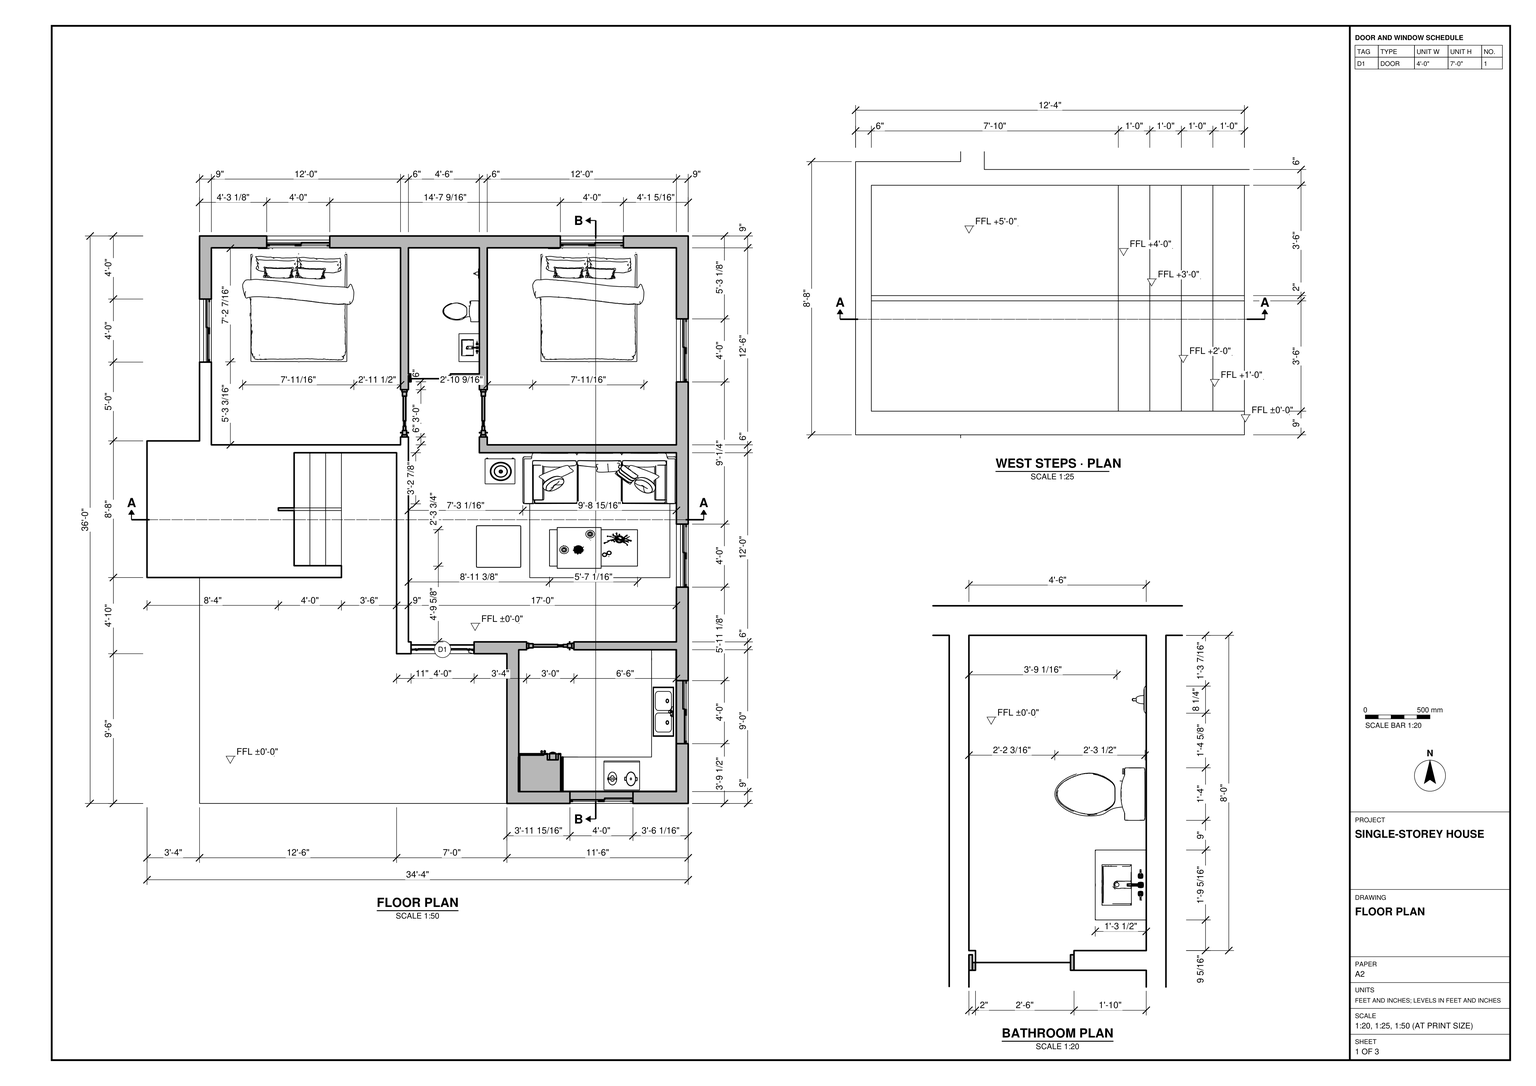
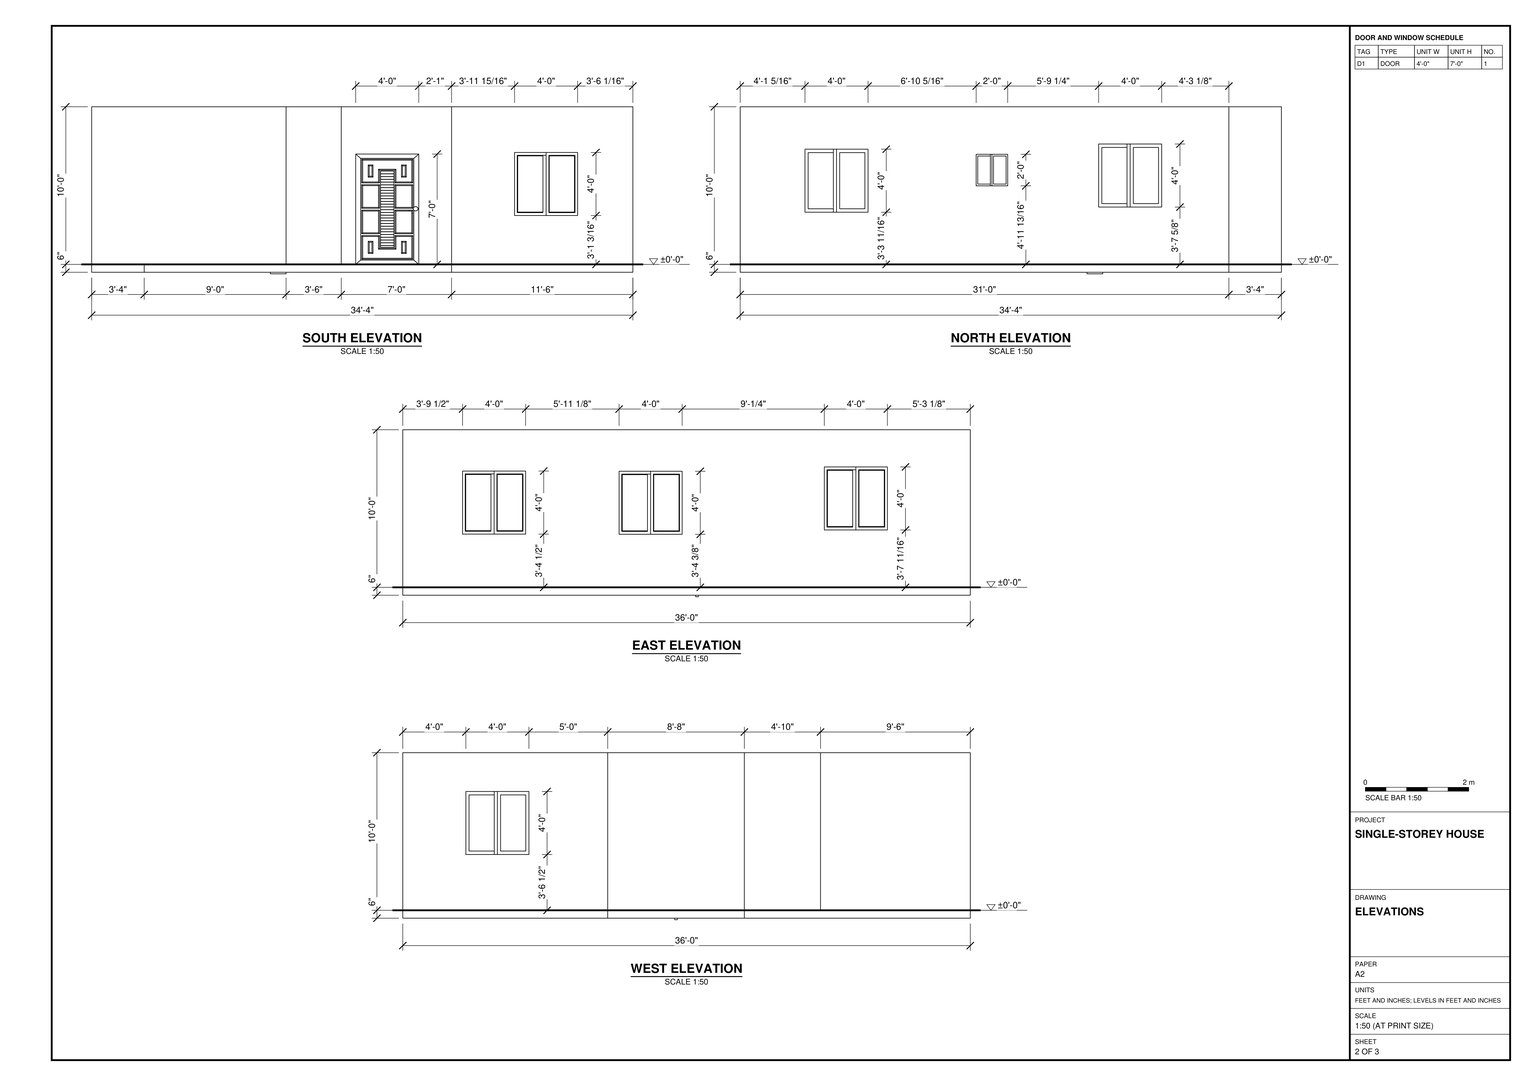
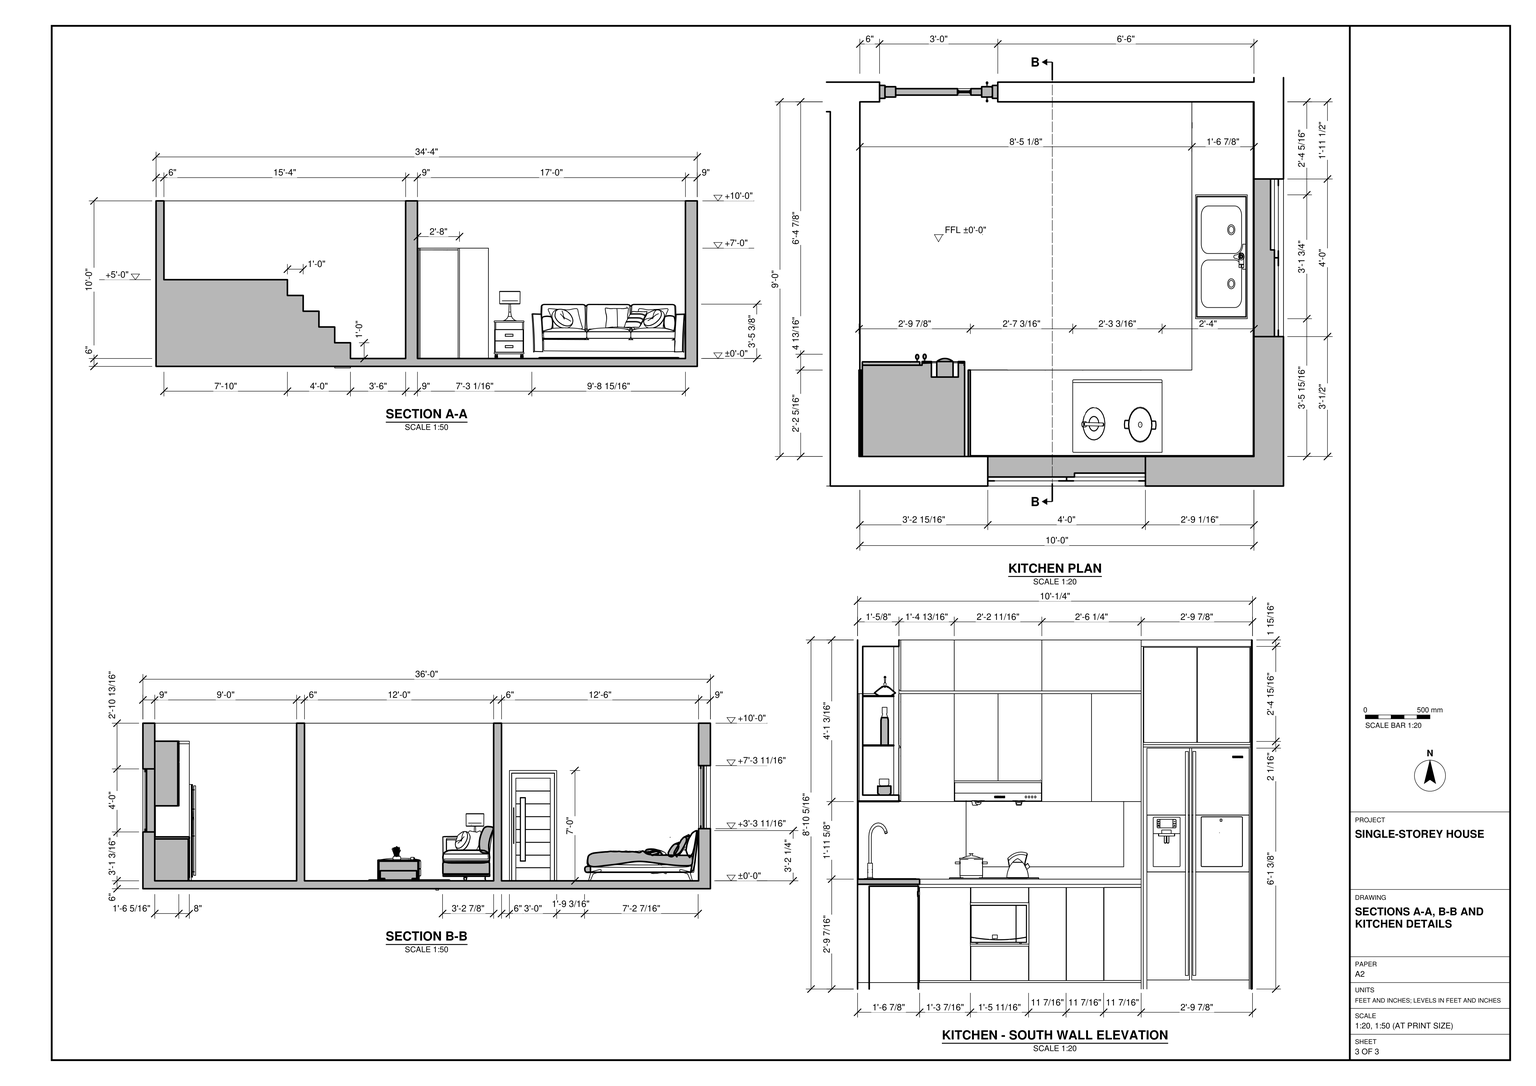
Build the house in SketchUp from task_files/diagram_01.pdf. Work in feet and inches. Set the finished floor of the single storey at ±0'-0". The overall model, including the west steps and floor slab, is 34'-4" east to west, 36'-0" north to south and 10'-7 3/16" high.

Follow the stepped footprint in the floor plan. Place the two bedrooms across the north end, with the narrow bathroom between them, the living room to the south and the kitchen projecting at the southeast corner. Model the 6" floor slab and use the wall thicknesses marked on the plan, including the 9" exterior walls and 6" partitions where indicated. Follow the level wall tops in the elevations. Use the enlarged west steps plan and section A-A to set out the raised landing and its flight down towards the house.

Fit the south entrance door and place the windows at the offsets and sill heights shown in the elevations. Position the beds, sofa and tables to match their plan footprints. Fit the bathroom toilet and vanity against the east wall. Use the kitchen detail views for the counters, lower and upper cabinets, sink, cooktop and refrigerator. Decor and loose items, including appliances, may be any suitable library components.

Keep shell elements and each furniture or joinery piece in separate groups or components, and use components for repeated parts. Save one SketchUp model as output_files/single_storey_house_with_west_steps_and_fitted_kitchen.skp.

# SketchUp Ruby script. Lengths in inches.
U = 1.inch
M = Sketchup.active_model
def pt(a) = Geom::Point3d.new(a.map { |v| v * U })
def face(e, loops, mat)
  f = e.add_face(loops[0].map { |a| pt(a) })
  loops[1..].each { |l| e.add_face(l.map { |a| pt(a) }).erase! }
  f.material = f.back_material = mat if mat
  f
end
# faces: each face lists its corners as indices into pts; further lists are holes
def faces(e, pts, list, mat = nil) = list.each { |f| face(e, (f[0].is_a?(Array) ? f : [f]).map { |l| l.map { |i| pts[i] } }, mat) }
# xy, xz, yz: faces in a plane at the given z, y or x. An outline is a flat list of corners, or four numbers for a rectangle; further outlines are holes
def ring(l) = l.size == 4 ? [[l[0], l[1]], [l[2], l[1]], [l[2], l[3]], [l[0], l[3]]] : l.each_slice(2).to_a
def flat(e, list, mat, &to3) = list.each { |f| face(e, (f[0].is_a?(Array) ? f : [f]).map { |l| ring(l).map { |u, v| to3.(u, v) } }, mat) }
def xy(e, z, list, mat = nil) = flat(e, list, mat) { |x, y| [x, y, z] }
def xz(e, y, list, mat = nil) = flat(e, list, mat) { |x, z| [x, y, z] }
def yz(e, x, list, mat = nil) = flat(e, list, mat) { |y, z| [x, y, z] }
def lines(e, pts, list) = list.each { |a, b| e.add_line(pt(pts[a]), pt(pts[b])) }
# prism: a flat outline (further loops are holes) pulled along v
def prism(e, loops, v, mat = nil)
  f = face(e, loops, mat); d = Geom::Vector3d.new(v.map { |x| x * U })
  f.pushpull(f.normal.samedirection?(d) ? d.length : -d.length)
end
def box(e, o, s, mat = nil) = prism(e, [[o, [o[0] + s[0], o[1], o[2]], [o[0] + s[0], o[1] + s[1], o[2]], [o[0], o[1] + s[1], o[2]]]], [0, 0, s[2]], mat)
def at(x, y, z, deg = 0) = Geom::Transformation.translation(pt([x, y, z])) * Geom::Transformation.rotation(ORIGIN, Z_AXIS, deg.degrees)
def axes(o, x, y, z) = Geom::Transformation.new([*x, 0, *y, 0, *z, 0, *pt(o).to_a, 1])
def part(name) = M.definitions.add(name)
# library, detail: a bought-in or finely detailed component or shape, given as its bounding box
def library(name, o, s) = part(name).tap { |d| box(d.entities, o, s) }
def detail(e, o, s) = box(e.add_group.entities, o, s)
def put(e, d, t, mat = nil) = e.add_instance(d, t).tap { |i| i.material = mat if mat }
def group(e, t, mat = nil) = e.add_group.tap { |g| g.transformation = t; g.material = mat if mat }.entities
root = M.entities
M.materials.add("Polis06_194").color = [79, 50, 36]
M.materials.add("[0012_Bisque]").color = [255, 228, 196]
M.materials.add("[Blacktop Old 02]").color = [143, 145, 145]
M.materials.add("[Carrera Marble]").color = [207, 207, 207]
M.materials.add("[Color M00]1").color = [255, 255, 255]
M.materials.add("[Color M05]").color = [100, 98, 98]
M.materials.add("[Color M07]").color = [46, 46, 46]
M.materials.add("[Color_001]").color = [226, 226, 226]
M.materials.add("[Field Square Tile]").color = [217, 201, 169]
M.materials.add("[Metal_Corrogated_Shiny]").color = [126, 127, 128]
M.materials.add("[Metal_Corrogated_Shiny]1").color = [193, 193, 193]
M.materials.add("[Translucent Glass Blue]").color = [100, 149, 237]
M.materials["[Translucent Glass Blue]"].alpha = 0.5
M.materials.add("[_0030_OldLace_]").color = [200, 200, 200]
M.materials.add("行者0155_1_1").color = [98, 90, 80]
c1 = library("devendra+jangid+[door]+drawings",[57.04,80.03,0],[48,84,6.66])
c2 = library("Спалня Венид",[0.07,-0.07,0],[84.71,86.8,39])
c3 = library("04+Sofa+y+Mesas (1)",[-94.93,-111.67,3.93],[153.81,110.61,64.28])
c4 = part("Janela aluminio")
xy(c4.entities,0,[[0,0,47.24,1.57],[23.62,1.57,47.24,2.76],[0,2.76,25.98,3.9375],[0,3.9375,47.24,5.91]])
xy(c4.entities,43.31,[[0,0,47.24,1.57],[23.62,1.57,47.24,2.76],[0,2.76,0,5.91,47.24,5.91,47.24,3.9375,25.98,3.9375,25.98,2.76],[25.98,2.76,47.24,3.9375]])
xz(c4.entities,1.57,[[0,0,23.62,0,23.62,41.34,21.26,41.34,21.26,1.97,1.97,1.97,1.97,41.34,23.62,41.34,23.62,43.31,0,43.31],[[23.62,0,47.24,43.31],[25.7,1.97,45.28,41.34]]])
xz(c4.entities,2.76,[[[0,0,23.62,43.31],[2.36,2.36,21.26,40.94]],[23.62,0,25.98,43.31]])
xz(c4.entities,2.76,[[2.36,2.36,21.26,40.94]],"[Translucent Glass Blue]")
xz(c4.entities,3.9375,[[25.98,0,25.98,2.36,44.88,2.36,44.88,40.94,25.98,40.94,25.98,43.31,47.24,43.31,47.24,0]])
xz(c4.entities,3.9375,[[25.98,2.36,44.88,40.94]],"[Translucent Glass Blue]")
yz(c4.entities,0,[[0,0,1.57,43.31],[2.76,0,5.91,43.31]])
yz(c4.entities,23.62,[[1.57,0,2.76,43.31]])
yz(c4.entities,25.98,[[2.76,0,3.9375,43.31]])
yz(c4.entities,47.24,[[0,0,1.57,43.31],[1.57,0,2.76,43.31],[3.9375,0,5.91,43.31]])
c5 = library("Framed entrance door",[0,0,0],[5.9375,43.31,84.65])
c6 = part("群组\#3")
xy(c6.entities,0,[[0,0,4.72,1.18],[0,34.25,4.72,35.43]],"Polis06_194")
xy(c6.entities,85.26,[[0,1.18,4.72,34.25]],"Polis06_194")
xy(c6.entities,86.61,[[0,0,4.72,35.43]],"Polis06_194")
xz(c6.entities,0,[[0,0,4.72,86.61]],"Polis06_194")
xz(c6.entities,1.18,[[0,0,2.36,85.26],[2.36,0,4.72,85.26]],"Polis06_194")
xz(c6.entities,34.25,[[0,0,4.72,85.26]],"Polis06_194")
xz(c6.entities,35.43,[[0,0,4.72,86.61]],"Polis06_194")
yz(c6.entities,0,[[0,0,1.18,86.61],[34.25,0,35.43,86.61],[1.18,85.26,34.25,86.61]],"Polis06_194")
yz(c6.entities,2.36,[[1.18,0,34.25,0,34.25,85.21,1.18,85.26]],"Polis06_194")
yz(c6.entities,4.72,[[0,0,1.18,86.61],[34.25,0,35.43,86.61],[1.18,85.26,34.25,86.61]],"Polis06_194")
c7 = library("TS396-4",[-0.02,-3.5,-3.5],[8.95,7,28.74])
c8 = library("K-3457 - Kohler Devonshire(R) elongated toilet with left-han",[-8.99,-6.22,0],[17.99,30.87,31.5])
c9 = library("30\" Kohler Jacquard Vanity",[0,0,0],[30,21.875,40.63])
c10 = part("Dishwasher5")
xy(c10.entities,0,[[0.39,0,29.13,23.62]],"[Metal_Corrogated_Shiny]")
xy(c10.entities,35.45,[[0.39,0,29.13,0.39]])
xy(c10.entities,35.49,[[0.39,0,29.13,0.39]])
xy(c10.entities,35.81,[[12.33,0,17.95,0.39]])
xy(c10.entities,37.36,[[12.33,0,17.95,0.39]])
xy(c10.entities,39.37,[[0.39,0,29.13,23.62]],"[Metal_Corrogated_Shiny]")
xz(c10.entities,-0.39,[[6.875,36.35,7.125,36.38,7.36,36.48,7.5625,36.63,7.72,36.84,7.82,37.08,7.86,37.34,7.83,37.59,7.74,37.84,7.59,38.05,7.39,38.21,7.16,38.32,6.91,38.35,6.66,38.33,6.43,38.23,6.22,38.07,6.06,37.87,5.96,37.63,5.93,37.375,5.95,37.11,6.05,36.87,6.2,36.66,6.39,36.5,6.625,36.39]],"[Metal_Corrogated_Shiny]1")
xz(c10.entities,0,[[0.39,0,29.13,35.45],[[0.39,35.49,29.13,39.37],[12.33,35.81,17.95,37.36],[6.875,36.35,6.625,36.39,6.39,36.5,6.2,36.66,6.05,36.87,5.95,37.11,5.93,37.375,5.96,37.63,6.06,37.87,6.22,38.07,6.43,38.23,6.66,38.33,6.91,38.35,7.16,38.32,7.39,38.21,7.59,38.05,7.74,37.84,7.83,37.59,7.86,37.34,7.82,37.08,7.72,36.84,7.5625,36.63,7.36,36.48,7.125,36.38]]])
xz(c10.entities,0.39,[[0.39,35.45,29.13,35.49],[12.33,35.81,17.95,37.36]])
xz(c10.entities,23.62,[[0.39,0,29.13,39.37]],"[Metal_Corrogated_Shiny]")
yz(c10.entities,0.39,[[0,0,0,35.45,0.39,35.45,0.39,35.49,0,35.49,0,39.37,23.62,39.37,23.62,0]],"[Metal_Corrogated_Shiny]")
yz(c10.entities,12.33,[[0,35.81,0.39,37.36]])
yz(c10.entities,17.95,[[0,35.81,0.39,37.36]])
yz(c10.entities,29.13,[[0,0,23.62,0,23.62,39.37,0,39.37,0,35.49,0.39,35.49,0.39,35.45,0,35.45]],"[Metal_Corrogated_Shiny]")
p = [[6.39,0,36.5],[6.625,0,36.39],[6.625,-0.39,36.39],[6.39,-0.39,36.5],[6.875,0,36.35],[6.875,-0.39,36.35],
  [7.125,0,36.38],[7.125,-0.39,36.38],[7.36,0,36.48],[7.36,-0.39,36.48],[6.2,0,36.66],[6.2,-0.39,36.66],
  [7.5625,0,36.63],[7.5625,-0.39,36.63],[7.72,0,36.84],[7.72,-0.39,36.84],[6.05,0,36.87],[6.05,-0.39,36.87],
  [7.82,0,37.08],[7.82,-0.39,37.08],[5.95,0,37.11],[5.95,-0.39,37.11],[5.93,0,37.375],[5.93,-0.39,37.375],
  [7.86,0,37.34],[7.86,-0.39,37.34],[7.83,0,37.59],[7.83,-0.39,37.59],[5.96,0,37.63],[5.96,-0.39,37.63],
  [6.06,0,37.87],[6.06,-0.39,37.87],[7.74,0,37.84],[7.74,-0.39,37.84],[7.59,0,38.05],[7.59,-0.39,38.05],
  [6.22,0,38.07],[6.22,-0.39,38.07],[7.39,0,38.21],[7.39,-0.39,38.21],[6.43,0,38.23],[6.43,-0.39,38.23],
  [6.66,0,38.33],[6.66,-0.39,38.33],[7.16,0,38.32],[7.16,-0.39,38.32],[6.91,0,38.35],[6.91,-0.39,38.35]]
faces(c10.entities,p,[[0,1,2,3],[1,4,5,2],[4,6,7,5],[6,8,9,7],[10,0,3,11],[8,12,13,9],[12,14,15,13],[16,10,11,17],
  [14,18,19,15],[20,16,17,21],[22,20,21,23],[18,24,25,19],[24,26,27,25],[28,22,23,29],[30,28,29,31],[26,32,33,27],
  [32,34,35,33],[36,30,31,37],[34,38,39,35],[40,36,37,41],[42,40,41,43],[38,44,45,39],[46,42,43,47],[44,46,47,45]],"[Metal_Corrogated_Shiny]1")
c11 = library("1",[-25.2,23.2,0],[33.86,19.68,25.36])
c12 = part("Cabinet panel \#1")
xy(c12.entities,0,[[0.6,0.08,0.63,16.59]],"行者0155_1_1")
xy(c12.entities,27.1,[[0.08,0.08,0.63,16.59]],"行者0155_1_1")
xz(c12.entities,0,[[0.52,0.08,0.63,0.08,0.63,27.02,0.08,27.02,0.08,0.53]],"行者0155_1_1")
xz(c12.entities,16.67,[[0.52,0.08,0.08,0.53,0.08,27.02,0.63,27.02,0.63,0.08]],"行者0155_1_1")
yz(c12.entities,0,[[0.08,0.61,16.59,27.02]],"行者0155_1_1")
yz(c12.entities,0.71,[[0.08,0.08,16.59,27.02]],"行者0155_1_1")
p = [[0.41,0.08,0.08],[0.6,0.08,0],[0.52,0,0.08],[0.63,0,0.08],[0.63,0.08,0],[0.71,0.08,0.08],
  [0.41,16.59,0.08],[0.6,16.59,0],[0.71,16.59,0.08],[0.63,16.59,0],[0.52,16.67,0.08],[0.63,16.67,0.08],
  [0.08,0.08,0.42],[0.08,0,0.53],[0.71,0.08,27.02],[0.63,0,27.02],[0.08,16.59,0.42],[0.08,16.67,0.53],
  [0.71,16.59,27.02],[0.63,16.67,27.02],[0,0.08,0.61],[0,16.59,0.61],[0,0.08,27.02],[0.08,0,27.02],
  [0,16.59,27.02],[0.08,16.67,27.02],[0.08,0.08,27.1],[0.63,0.08,27.1],[0.08,16.59,27.1],[0.63,16.59,27.1]]
faces(c12.entities,p,[[0,1,2],[3,2,1,4],[4,5,3],[0,6,7,1],[8,5,4,9],[7,6,10],[10,11,9,7],[8,9,11],
  [12,0,2,13],[5,14,15,3],[0,12,16,6],[6,16,17,10],[18,8,11,19],[20,12,13],[16,12,20,21],[16,21,17],
  [22,20,13,23],[21,24,25,17],[26,22,23],[27,26,23,15],[14,27,15],[26,28,24,22],[29,27,14,18],[24,28,25],
  [28,29,19,25],[29,18,19]],"行者0155_1_1")
c13 = library("Range hood",[0,0.31,0],[20.46,27.69,6.07])
c14 = part("Component\#6")
prism(c14.entities,[[[0,0,0],[0,0,28.41],[0,0.53,28.9375],[0,0.71,28.9375],[0,0.71,0]]],[17.47,0,0],"行者0155_1_1")
c15 = part("Cabinet panel \#2")
xy(c15.entities,0,[[0.63,0.079,0.641,18.822]],"行者0155_1_1")
xy(c15.entities,32.864,[[0.079,0.079,0.63,18.822]],"行者0155_1_1")
xz(c15.entities,0,[[0.5625,0.079,0.63,0.079,0.63,32.786,0.079,32.786,0.079,0.5625]],"行者0155_1_1")
xz(c15.entities,18.9,[[0.5625,0.079,0.079,0.5625,0.079,32.786,0.63,32.786,0.63,0.079]],"行者0155_1_1")
yz(c15.entities,0,[[0.079,0.641,18.822,32.786]],"行者0155_1_1")
yz(c15.entities,0.709,[[0.079,0.079,18.822,32.786]],"行者0155_1_1")
p = [[0.633,0.079,0.003],[0.641,0.079,0],[0.63,0.068,0.011],[0.5625,0,0.079],[0.451,0.079,0.079],[0.63,0.079,0],
  [0.63,0,0.079],[0.709,0.079,0.079],[0.641,18.822,0],[0.451,18.822,0.079],[0.633,18.822,0.003],[0.63,18.822,0],
  [0.709,18.822,0.079],[0.63,18.833,0.011],[0.5625,18.9,0.079],[0.63,18.9,0.079],[0.079,0.079,0.451],[0.079,0,0.5625],
  [0.709,0.079,32.786],[0.63,0,32.786],[0.079,18.822,0.451],[0.079,18.9,0.5625],[0.709,18.822,32.786],[0.63,18.9,32.786],
  [0,0.079,0.641],[0,18.822,0.641],[0,0.079,32.786],[0.079,0,32.786],[0,18.822,32.786],[0.079,18.9,32.786],
  [0.079,0.079,32.864],[0.63,0.079,32.864],[0.079,18.822,32.864],[0.63,18.822,32.864]]
faces(c15.entities,p,[[0,1,2,3,4],[1,5,2,6,3,2],[5,0,7,6,2],[8,1,0,4,9,10],[5,11,10,12,7,0],[13,8,10,9,14],[10,11,13,15,12],[11,8,13,14,15,13],
  [16,4,3,17],[7,18,19,6],[16,20,9,4],[21,14,9,20],[22,12,15,23],[24,16,17],[20,16,24,25],[20,25,21],
  [26,24,17,27],[25,28,29,21],[30,26,27],[31,30,27,19],[18,31,19],[30,32,28,26],[33,31,18,22],[28,32,29],
  [32,33,23,29],[33,22,23]],"行者0155_1_1")
c16 = part("Cabinet panel \#3")
xy(c16.entities,0,[[0.6,0.08,0.63,16.59]],"行者0155_1_1")
xy(c16.entities,27.1,[[0.08,0.08,0.63,16.59]],"行者0155_1_1")
xz(c16.entities,0,[[0.52,0.08,0.63,0.08,0.63,27.02,0.08,27.02,0.08,0.53]],"行者0155_1_1")
xz(c16.entities,16.67,[[0.52,0.08,0.08,0.53,0.08,27.02,0.63,27.02,0.63,0.08]],"行者0155_1_1")
yz(c16.entities,0,[[0.08,0.61,16.59,27.02]],"行者0155_1_1")
yz(c16.entities,0.71,[[0.08,0.08,16.59,27.02]],"行者0155_1_1")
p = [[0.41,0.08,0.08],[0.6,0.08,0],[0.52,0,0.08],[0.63,0,0.08],[0.63,0.08,0],[0.71,0.08,0.08],
  [0.41,16.59,0.08],[0.6,16.59,0],[0.71,16.59,0.08],[0.63,16.59,0],[0.52,16.67,0.08],[0.63,16.67,0.08],
  [0.08,0.08,0.42],[0.08,0,0.53],[0.71,0.08,27.02],[0.63,0,27.02],[0.08,16.59,0.42],[0.08,16.67,0.53],
  [0.71,16.59,27.02],[0.63,16.67,27.02],[0,0.08,0.61],[0,16.59,0.61],[0,0.08,27.02],[0.08,0,27.02],
  [0,16.59,27.02],[0.08,16.67,27.02],[0.08,0.08,27.1],[0.63,0.08,27.1],[0.08,16.59,27.1],[0.63,16.59,27.1]]
faces(c16.entities,p,[[0,1,2],[3,2,1,4],[4,5,3],[0,6,7,1],[8,5,4,9],[7,6,10],[10,11,9,7],[8,9,11],
  [12,0,2,13],[5,14,15,3],[0,12,16,6],[6,16,17,10],[18,8,11,19],[20,12,13],[16,12,20,21],[16,21,17],
  [22,20,13,23],[21,24,25,17],[26,22,23],[27,26,23,15],[14,27,15],[26,28,24,22],[29,27,14,18],[24,28,25],
  [28,29,19,25],[29,18,19]],"行者0155_1_1")
c17 = part("Component\#35")
xy(c17.entities,0,[[1.261,0.63,20.265,0.641]],"行者0155_1_1")
xy(c17.entities,32.864,[[1.261,0.079,20.265,0.63]],"行者0155_1_1")
xz(c17.entities,0,[[1.261,0.641,20.265,32.786]],"行者0155_1_1")
xz(c17.entities,0.709,[[1.261,0.079,20.265,32.786]],"行者0155_1_1")
yz(c17.entities,1.181,[[0.5625,0.079,0.079,0.5625,0.079,32.786,0.63,32.786,0.63,0.079]],"行者0155_1_1")
yz(c17.entities,20.345,[[0.5625,0.079,0.63,0.079,0.63,32.786,0.079,32.786,0.079,0.5625]],"行者0155_1_1")
p = [[1.25,0.63,0.011],[1.261,0.641,0],[1.261,0.633,0.003],[1.261,0.451,0.079],[1.181,0.5625,0.079],[20.265,0.641,0],
  [20.265,0.633,0.003],[20.265,0.451,0.079],[20.276,0.63,0.011],[20.345,0.5625,0.079],[1.261,0.63,0],[1.181,0.63,0.079],
  [1.261,0.709,0.079],[20.265,0.63,0],[20.265,0.709,0.079],[20.345,0.63,0.079],[1.181,0.079,0.5625],[1.261,0.079,0.451],
  [20.265,0.079,0.451],[20.345,0.079,0.5625],[1.261,0.709,32.786],[1.181,0.63,32.786],[20.265,0.709,32.786],[20.345,0.63,32.786],
  [1.261,0,0.641],[20.265,0,0.641],[1.261,0,32.786],[1.181,0.079,32.786],[20.265,0,32.786],[20.345,0.079,32.786],
  [1.261,0.079,32.864],[20.265,0.079,32.864],[1.261,0.63,32.864],[20.265,0.63,32.864]]
faces(c17.entities,p,[[0,1,2,3,4],[1,5,6,7,3,2],[6,5,8,9,7],[10,1,0,4,11,0],[2,10,0,11,12],[13,10,2,12,14,6],[5,13,8,15,9,8],[13,6,14,15,8],
  [16,4,3,17],[18,17,3,7],[18,7,9,19],[20,12,11,21],[14,22,23,15],[17,24,16],[17,18,25,24],[25,18,19],
  [24,26,27,16],[28,25,19,29],[26,30,27],[31,30,26,28],[31,28,29],[30,32,21,27],[33,31,29,23],[32,20,21],
  [32,33,22,20],[22,33,23]],"行者0155_1_1")
c18 = library("Cooktop with cookware",[0,0,0],[27.875,16.26,6.75])
c19 = library("Group\#39",[0,1.25,-0.39],[21.22,17.8,11.81])
c20 = library("Group\#43",[0,0,0],[0.71,19.52,28.35])
c21 = library("Group\#44",[0,0,0],[0.71,12.75,28.35])
c22 = library("Group\#7",[0,0,0],[37.83,27.94,106.3])
c23 = library("Group\#40",[0,0,0],[0.71,12.75,28.35])
c24 = library("Group\#36",[0,0,-0.15],[0.71,21.95,10.47])
c25 = library("Group\#42",[0,0,-0.15],[0.71,21.95,4.61])
c26 = library("Group\#51",[0,0,0],[32.28,11.75,25.51])
c27 = library("Group\#33",[0,0,0],[24.33,15.75,49.21])
xy(root,-1.1875,[[136,223,148,225]])
xy(root,0,[[40,0,40,172,0,172,0,276,40,276,40,432,412,432,412,0]])
xy(root,6,[[40,0,274,0,274,114,190,114,190,267,148,267,148,172,40,172]],"[Carrera Marble]")
xy(root,6,[[283,9,403,9,403,117,325,117,325,123,403,123,403,267,253,267,253,279,259,279,259,273,403,273,403,423,259,423,259,315,253,315,253,321,231,321,231,327,253,327,253,423,199,423,199,327,201,327,201,321,199,321,199,315,193,315,193,423,49,423,49,273,193,273,193,279,199,279,199,123,201,123,201,114,249,114,249,123,289,123,289,117,283,117]],"[Field Square Tile]")
xy(root,18,[[124,223,136,225]])
xy(root,18,[[136,181,148,223],[136,225,148,267]],"[Carrera Marble]")
xy(root,30,[[112,223,124,225]])
xy(root,30,[[124,181,136,223],[124,225,136,267]],"[Carrera Marble]")
xy(root,42,[[100,223,112,225]])
xy(root,42,[[112,181,124,223],[112,225,124,267]],"[Carrera Marble]")
xy(root,43.21,[[321.95,0,369.95,9]])
xy(root,45.71,[[314.68,423,362.68,432]])
xy(root,46.39,[[403,164.67,412,212.67]])
xy(root,46.52,[[403,45.51,412,93.51]])
xy(root,48.47,[[40,335.98,49,383.98]])
xy(root,49.65,[[91.13,423,139.13,432]])
xy(root,49.68,[[403,320.9,412,368.9]])
xy(root,54,[[6,223,100,225]])
xy(root,54,[[100,181,112,223],[100,225,112,267]],"[Carrera Marble]")
xy(root,65.81,[[208.37,423,232.37,432]])
xy(root,66,[[6,181,100,223],[6,225,100,267]],"[Carrera Marble]")
xy(root,89.81,[[208.37,423,232.37,432]])
xy(root,90,[[201,114,249,123],[289,117,325,123],[193,279,199,315],[253,279,259,315],[201,321,231,327]])
xy(root,91.21,[[321.95,0,369.95,9]])
xy(root,93.71,[[314.68,423,362.68,432]])
xy(root,94.39,[[403,164.67,412,212.67]])
xy(root,94.52,[[403,45.51,412,93.51]])
xy(root,96.47,[[40,335.98,49,383.98]])
xy(root,97.65,[[91.13,423,139.13,432]])
xy(root,97.68,[[403,320.9,412,368.9]])
xy(root,126,[[[274,0,412,0,412,432,40,432,40,276,0,276,0,172,148,172,148,181,6,181,6,267,190,267,190,114,274,114],[199,123,403,267],[49,273,193,423],[259,273,403,423],[283,9,403,117],[199,327,253,423],[199,279,253,321]]],"[0012_Bisque]")
xz(root,0,[[40,0,274,6]])
xz(root,0,[[[274,0,412,126],[321.95,43.21,369.95,91.21]]],"[Blacktop Old 02]")
xz(root,9,[[[283,6,403,126],[321.95,43.21,369.95,91.21]]],"[0012_Bisque]")
xz(root,45.51,[[403,46.52,412,94.52]])
xz(root,93.51,[[403,46.52,412,94.52]])
xz(root,114,[[190,6,201,6,201,90,249,90,249,6,274,6,274,126,190,126]],"[0012_Bisque]")
xz(root,117,[[283,6,289,6,289,90,325,90,325,6,403,6,403,126,283,126]],"[0012_Bisque]")
xz(root,123,[[199,6,199,126,403,126,403,6,325,6,325,90,289,90,289,6,249,6,249,90,201,90,201,6]],"[0012_Bisque]")
xz(root,164.67,[[403,46.39,412,94.39]])
xz(root,172,[[0,0,40,0,40,6,148,6,148,126,0,126]],"[Blacktop Old 02]")
xz(root,181,[[136,18,136,30,124,30,124,42,112,42,112,54,100,54,100,66,6,66,6,126,148,126,148,18]],"[Blacktop Old 02]")
xz(root,212.67,[[403,46.39,412,94.39]])
xz(root,223,[[136,-1.1875,148,18],[124,18,136,30],[112,30,124,42],[100,42,112,54],[6,54,100,66]])
xz(root,225,[[136,-1.1875,148,18],[124,18,136,30],[112,30,124,42],[100,42,112,54],[6,54,100,66]])
xz(root,267,[[190,90,199,126]])
xz(root,267,[[253,6,403,6,403,126,199,126,199,90,253,90]],"[0012_Bisque]")
xz(root,267,[[148,6,190,6,190,126,6,126,6,66,100,66,100,54,112,54,112,42,124,42,124,30,136,30,136,18,148,18]],"[Blacktop Old 02]")
xz(root,273,[[49,6,193,126],[259,6,403,126]],"[0012_Bisque]")
xz(root,276,[[0,0,40,126]],"[Blacktop Old 02]")
xz(root,279,[[193,6,199,90],[253,6,259,90]])
xz(root,279,[[199,90,253,126]],"[0012_Bisque]")
xz(root,315,[[193,6,199,90],[253,6,259,90]])
xz(root,320.9,[[403,49.68,412,97.68]])
xz(root,321,[[199,6,201,6,201,90,231,90,231,6,253,6,253,126,199,126]],"[0012_Bisque]")
xz(root,327,[[199,6,199,126,253,126,253,6,231,6,231,90,201,90,201,6]],"[0012_Bisque]")
xz(root,335.98,[[40,48.47,49,96.47]])
xz(root,368.9,[[403,49.68,412,97.68]])
xz(root,383.98,[[40,48.47,49,96.47]])
xz(root,423,[[[49,6,193,126],[91.13,49.65,139.13,97.65]],[[199,6,253,126],[208.37,65.81,232.37,89.81]],[[259,6,403,126],[314.68,45.71,362.68,93.71]]],"[0012_Bisque]")
xz(root,432,[[[40,0,412,126],[314.68,45.71,362.68,93.71],[91.13,49.65,139.13,97.65],[208.37,65.81,232.37,89.81]]],"[Blacktop Old 02]")
yz(root,0,[[172,0,276,126]],"[Blacktop Old 02]")
yz(root,6,[[223,54,225,54,225,66,267,66,267,126,181,126,181,66,223,66]],"[Blacktop Old 02]")
yz(root,40,[[0,0,172,6]])
yz(root,40,[[[276,0,432,126],[335.98,48.47,383.98,96.47]]],"[Blacktop Old 02]")
yz(root,49,[[[273,6,423,126],[335.98,48.47,383.98,96.47]]],"[0012_Bisque]")
yz(root,91.13,[[423,49.65,432,97.65]])
yz(root,100,[[223,42,225,54],[181,54,223,66],[225,54,267,66]])
yz(root,112,[[223,30,225,42],[181,42,223,54],[225,42,267,54]])
yz(root,124,[[223,18,225,30],[181,30,223,42],[225,30,267,42]])
yz(root,136,[[223,-1.1875,225,18],[181,18,223,30],[225,18,267,30]])
yz(root,139.13,[[423,49.65,432,97.65]])
yz(root,148,[[223,-1.1875,225,6],[181,6,223,18],[225,6,267,18]])
yz(root,148,[[172,6,181,126]],"[Blacktop Old 02]")
yz(root,190,[[114,6,267,126]],"[Blacktop Old 02]")
yz(root,193,[[273,6,273,126,423,126,423,6,315,6,315,90,279,90,279,6]],"[0012_Bisque]")
yz(root,199,[[123,6,279,6,279,90,267,90,267,126,123,126],[315,6,321,6,321,126,279,126,279,90,315,90],[327,6,423,126]],"[0012_Bisque]")
yz(root,201,[[114,6,123,90]])
yz(root,201,[[321,6,327,90]],"[0012_Bisque]")
yz(root,208.37,[[423,65.81,432,89.81]])
yz(root,231,[[321,6,327,90]])
yz(root,232.37,[[423,65.81,432,89.81]])
yz(root,249,[[114,6,123,90]])
yz(root,253,[[267,6,279,90],[315,6,315,90,279,90,279,126,321,126,321,6],[327,6,423,126]],"[0012_Bisque]")
yz(root,259,[[273,6,279,6,279,90,315,90,315,6,423,6,423,126,273,126]],"[0012_Bisque]")
yz(root,274,[[0,6,114,126]],"[0012_Bisque]")
yz(root,283,[[9,6,117,126]],"[0012_Bisque]")
yz(root,289,[[117,6,123,90]])
yz(root,314.68,[[423,45.71,432,93.71]])
yz(root,321.95,[[0,43.21,9,91.21]])
yz(root,325,[[117,6,123,90]])
yz(root,362.68,[[423,45.71,432,93.71]])
yz(root,369.95,[[0,43.21,9,91.21]])
yz(root,403,[[[9,6,117,126],[45.51,46.52,93.51,94.52]],[[123,6,267,126],[164.67,46.39,212.67,94.39]],[[273,6,423,126],[320.9,49.68,368.9,97.68]]],"[0012_Bisque]")
yz(root,412,[[[0,0,432,126],[45.51,46.52,93.51,94.52],[164.67,46.39,212.67,94.39],[320.9,49.68,368.9,97.68]]],"[Blacktop Old 02]")
p = [[197.94,281.69,0],[199,279,6]]
lines(root,p,[[0,1]])
put(root,c1,axes([143.96,120.66,-74.03],[1,0,0],[0,0,1],[0,-1,0]))
put(root,c2,at(293.51,336.27,6))
put(root,c3,axes([344.71,267.91,2.07],[0.99,0,0],[0,0.86,0],[0,0,1]))
put(root,c2,at(72.69,336.27,6),"[0012_Bisque]")
put(root,c4,axes([314.68,423,45.71],[1.016,0,0],[0,1,0],[0,0,1.10836]))
put(root,c5,axes([193.0625,279,6],[1,0,0],[0,0.83127,0],[0,0,0.99237]))
put(root,c6,axes([199,325.72,6],[0,-1,0],[0.90311,0,0],[0,0,0.96982]))
put(root,c5,axes([253.0625,279,6],[1,0,0],[0,0.83127,0],[0,0,0.99237]),"[0012_Bisque]")
put(root,c5,axes([325,117.0625,6],[0,1,0],[-0.83127,0,0],[0,0,0.99237]))
put(root,c7,axes([252.99,403.41,41.49],[-1,0,0],[0,1.1793,0],[0,0,1.85]))
put(root,c8,axes([247.1,374.66,6],[0,0.89,0],[-0.89,0,0],[0,0,0.89]))
put(root,c9,axes([237.47,357.625,6],[0,-0.71,0],[0.71,0,0],[0,0,0.71]))
put(root,c4,axes([91.13,423,49.65],[1.016,0,0],[0,1,0],[0,0,1.10836]))
put(root,c4,axes([412,320.9,49.68],[0,1.016,0],[-1,0,0],[0,0,1.10836]))
put(root,c4,axes([412,164.67,46.39],[0,1.016,0],[-1,0,0],[0,0,1.10836]))
put(root,c4,axes([49,335.98,48.47],[0,1.016,0],[-1,0,0],[0,0,1.10836]))
put(root,c4,axes([208.37,426.09,65.81],[0.508,0,0],[0,1,0],[0,0,0.55418]))
put(root,c4,axes([321.95,0,43.21],[1.016,0,0],[0,1,0],[0,0,1.10836]))
put(root,c4,axes([412,45.51,46.52],[0,1.016,0],[-1,0,0],[0,0,1.10836]))
g1 = group(root,at(282.75,9,6))
put(g1,c10,axes([101.68,106.96,0],[0,-0.88623,0],[0.63632,0,0],[0,0,0.7954]))
put(g1,c11,axes([136.78,70.04,25.24],[0,1.1142,0],[-0.8,0,0],[0,0,1]),"[Color_001]")
put(g1,c12,axes([90.8125,17.55,63.39],[0,1.1142,0],[-0.8,0,0],[0,0,0.9801]))
put(g1,c13,axes([64,23.83,55.96],[0,-1.15353,0],[0.952,0,0],[0,0,1.19]))
put(g1,c14,axes([101.92,61.43,1.97],[0,1.1142,0],[-0.8,0,0],[0,0,1]))
put(g1,c15,axes([64.14,17.55,57.09],[0,1.1142,0],[-0.8,0,0],[0,0,1]))
put(g1,c16,axes([77.47,17.55,63.39],[0,1.1142,0],[-0.8,0,0],[0,0,0.9801]))
put(g1,c14,axes([101.92,41.96,1.97],[0,1.1142,0],[-0.8,0,0],[0,0,1]))
put(g1,c17,axes([32.96,17.55,57.09],[0.78901,0,0],[0,1.1142,0],[0,0,1]))
put(g1,c18,axes([92.28,23.36,33.46],[-0.976,0,0],[0,-1.35932,0],[0,0,1.22]),"[Color M00]1")
g2 = group(g1,at(77.88,17.55,90.77))
xy(g2,0,[[12.993,0.702,29.143,0.708]],"行者0155_1_1")
xy(g2,15.531,[[12.993,0.088,29.143,0.702]],"行者0155_1_1")
xz(g2,0,[[12.993,0.635,29.143,15.452]],"行者0155_1_1")
xz(g2,0.79,[[12.993,0.079,29.143,15.452]],"行者0155_1_1")
yz(g2,12.93,[[0.62,0.079,0.088,0.556,0.088,15.452,0.702,15.452,0.702,0.079]],"行者0155_1_1")
yz(g2,29.206,[[0.62,0.079,0.702,0.079,0.702,15.452,0.088,15.452,0.088,0.556]],"行者0155_1_1")
p = [[12.993,0.708,0],[12.993,0.704,0.002],[12.993,0.496,0.079],[12.93,0.62,0.079],[12.989,0.702,0.005],[29.143,0.496,0.079],
  [29.143,0.708,0],[29.143,0.704,0.002],[29.147,0.702,0.005],[29.206,0.62,0.079],[12.93,0.702,0.079],[12.993,0.702,0],
  [29.143,0.702,0],[29.206,0.702,0.079],[12.993,0.79,0.079],[29.143,0.79,0.079],[12.993,0.088,0.445],[12.93,0.088,0.556],
  [29.143,0.088,0.445],[29.206,0.088,0.556],[12.993,0.79,15.452],[12.93,0.702,15.452],[29.206,0.702,15.452],[29.143,0.79,15.452],
  [12.993,0,0.635],[29.143,0,0.635],[12.93,0.088,15.452],[12.993,0,15.452],[29.206,0.088,15.452],[29.143,0,15.452],
  [12.993,0.088,15.531],[29.143,0.088,15.531],[12.993,0.702,15.531],[29.143,0.702,15.531]]
faces(g2,p,[[0,1,2,3,4],[5,2,1,0,6,7],[7,6,8,9,5],[3,10,4,11,0,4],[6,12,8,13,9,8],[1,11,4,10,14],[12,11,1,14,15,7],[8,12,7,15,13],
  [2,16,17,3],[18,16,2,5],[18,5,9,19],[20,14,10,21],[22,13,15,23],[17,16,24],[16,18,25,24],[18,19,25],
  [26,17,24,27],[19,28,29,25],[30,26,27],[31,30,27,29],[28,31,29],[30,32,21,26],[33,31,28,22],[32,20,21],
  [32,33,23,20],[33,22,23]],"行者0155_1_1")
put(g1,c19,axes([85.76,27.57,14.14],[-0.8,0,0],[0,-1.1142,0],[0,0,1]))
put(g1,c20,axes([101.36,25.53,2.56],[0,1.1142,0],[-0.792,0,0],[0,0,1]))
g3 = group(g1,at(107.66,-0.46,90.77))
xy(g3,0,[[-0.5,18.1,-0.46,40.59]],"行者0155_1_1")
xy(g3,15.53,[[-0.5,18.1,-0.0625,40.59]],"行者0155_1_1")
xz(g3,18.01,[[-0.5,0.08,-0.4,0.08,-0.0625,0.5,-0.0625,15.45,-0.5,15.45]],"行者0155_1_1")
xz(g3,40.68,[[-0.5,0.08,-0.5,15.45,-0.0625,15.45,-0.0625,0.5,-0.4,0.08]],"行者0155_1_1")
yz(g3,-0.57,[[18.1,0.08,40.59,15.45]],"行者0155_1_1")
yz(g3,0,[[18.1,0.58,40.59,15.45]],"行者0155_1_1")
p = [[-0.57,18.1,0.08],[-0.5,18.1,0],[-0.5,18.01,0.08],[-0.46,18.1,0],[-0.4,18.01,0.08],[-0.31,18.1,0.08],
  [-0.5,40.59,0],[-0.57,40.59,0.08],[-0.46,40.59,0],[-0.31,40.59,0.08],[-0.5,40.68,0.08],[-0.4,40.68,0.08],
  [-0.57,18.1,15.45],[-0.5,18.01,15.45],[-0.0625,18.01,0.5],[-0.0625,18.1,0.39],[-0.0625,40.59,0.39],[-0.5,40.68,15.45],
  [-0.57,40.59,15.45],[-0.0625,40.68,0.5],[0,18.1,0.58],[0,40.59,0.58],[-0.0625,18.01,15.45],[0,18.1,15.45],
  [-0.0625,40.68,15.45],[0,40.59,15.45],[-0.5,18.1,15.53],[-0.0625,18.1,15.53],[-0.5,40.59,15.53],[-0.0625,40.59,15.53]]
faces(g3,p,[[0,1,2],[1,3,4,2],[4,3,5],[6,1,0,7],[3,8,9,5],[10,6,7],[8,6,10,11],[9,8,11],
  [12,0,2,13],[14,4,5,15],[5,9,16,15],[17,10,7,18],[16,9,11,19],[14,15,20],[15,16,21,20],[16,19,21],
  [22,14,20,23],[19,24,25,21],[26,12,13],[27,26,13,22],[27,22,23],[26,28,18,12],[29,27,23,25],[28,17,18],
  [28,29,24,17],[24,29,25]],"行者0155_1_1")
g4 = group(g1,at(107.66,40.4,90.77))
xy(g4,0,[[-0.5,0.09,-0.48,40.18]],"行者0155_1_1")
xy(g4,15.53,[[-0.5,0.09,-0.0625,40.18]],"行者0155_1_1")
xz(g4,0,[[-0.5,0.08,-0.42,0.08,-0.0625,0.52,-0.0625,15.45,-0.5,15.45]],"行者0155_1_1")
xz(g4,40.27,[[-0.5,0.08,-0.5,15.45,-0.0625,15.45,-0.0625,0.52,-0.42,0.08]],"行者0155_1_1")
yz(g4,-0.57,[[0.09,0.08,40.18,15.45]],"行者0155_1_1")
yz(g4,0,[[0.09,0.6,40.18,15.45]],"行者0155_1_1")
p = [[-0.57,0.09,0.08],[-0.5,0.09,0],[-0.5,0,0.08],[-0.48,0.09,0],[-0.33,0.09,0.08],[-0.42,0,0.08],
  [-0.5,40.18,0],[-0.57,40.18,0.08],[-0.33,40.18,0.08],[-0.48,40.18,0],[-0.5,40.27,0.08],[-0.42,40.27,0.08],
  [-0.57,0.09,15.45],[-0.5,0,15.45],[-0.0625,0.09,0.41],[-0.0625,0,0.52],[-0.0625,40.18,0.41],[-0.5,40.27,15.45],
  [-0.57,40.18,15.45],[-0.0625,40.27,0.52],[0,0.09,0.6],[0,40.18,0.6],[-0.0625,0,15.45],[0,0.09,15.45],
  [-0.0625,40.27,15.45],[0,40.18,15.45],[-0.5,0.09,15.53],[-0.0625,0.09,15.53],[-0.5,40.18,15.53],[-0.0625,40.18,15.53]]
faces(g4,p,[[0,1,2],[3,4,5],[5,2,1,3],[6,1,0,7],[8,4,3,9],[10,6,7],[8,9,11],[9,6,10,11],
  [12,0,2,13],[4,14,15,5],[4,8,16,14],[17,10,7,18],[16,8,11,19],[15,14,20],[14,16,21,20],[16,19,21],
  [22,15,20,23],[19,24,25,21],[26,12,13],[27,26,13,22],[27,22,23],[26,28,18,12],[29,27,23,25],[28,17,18],
  [28,29,24,17],[24,29,25]],"行者0155_1_1")
put(g1,c21,axes([56.64,25.53,2.56],[0,1.1142,0],[-0.88776,0,0],[0,0,1]))
put(g1,c22,axes([0,0,0],[0.896,0,0],[0,1.1142,0],[0,0,1]))
put(g1,c23,axes([68.08,25.53,2.56],[0,1.1142,0],[-0.88776,0,0],[0,0,1]))
g5 = group(g1,at(34.93,17.55,90.77))
xy(g5,0,[[-0.97,0.7,29.14,0.74]],"行者0155_1_1")
xy(g5,15.53,[[-0.97,0.09,29.14,0.7]],"行者0155_1_1")
xz(g5,0,[[-0.97,0.52,29.14,15.45]],"行者0155_1_1")
xz(g5,0.79,[[-0.97,0.08,29.14,15.45]],"行者0155_1_1")
yz(g5,-1.03,[[0.625,0.08,0.09,0.46,0.09,15.45,0.7,15.45,0.7,0.08]],"行者0155_1_1")
yz(g5,29.21,[[0.625,0.08,0.7,0.08,0.7,15.45,0.09,15.45,0.09,0.46]],"行者0155_1_1")
p = [[-0.97,0.74,0],[-0.97,0.71,0.01],[-0.97,0.48,0.08],[-1.03,0.625,0.08],[-0.99,0.7,0.02],[29.14,0.48,0.08],
  [29.14,0.74,0],[29.14,0.71,0.01],[29.16,0.7,0.02],[29.21,0.625,0.08],[-1.03,0.7,0.08],[-0.97,0.7,0],
  [29.14,0.7,0],[29.21,0.7,0.08],[-0.97,0.79,0.08],[29.14,0.79,0.08],[-0.97,0.09,0.36],[29.14,0.09,0.36],
  [-1.03,0.09,0.46],[29.21,0.09,0.46],[-0.97,0.79,15.45],[-1.03,0.7,15.45],[29.14,0.79,15.45],[29.21,0.7,15.45],
  [29.14,0,0.52],[-0.97,0,0.52],[-0.97,0,15.45],[-1.03,0.09,15.45],[29.14,0,15.45],[29.21,0.09,15.45],
  [29.14,0.09,15.53],[-0.97,0.09,15.53],[-0.97,0.7,15.53],[29.14,0.7,15.53]]
faces(g5,p,[[0,1,2,3,4],[5,2,1,0,6,7],[7,6,8,9,5],[3,10,4,11,0,4],[6,12,8,13,9,8],[12,11,1,14,15,7],[1,11,4,10,14],[12,7,15,13,8],
  [16,2,5,17],[2,16,18,3],[17,5,9,19],[20,14,10,21],[15,22,23,13],[16,17,24,25],[16,25,18],[24,17,19],
  [25,26,27,18],[28,24,19,29],[30,31,26,28],[26,31,27],[30,28,29],[31,32,21,27],[33,30,29,23],[32,33,22,20],
  [32,20,21],[22,33,23]],"行者0155_1_1")
g6 = group(g1,at(61.61,17.55,90.77))
xy(g6,0,[[2.59,0.69,29.14,0.7]],"行者0155_1_1")
xy(g6,15.53,[[2.59,0.09,29.14,0.7]],"行者0155_1_1")
xz(g6,0,[[2.59,0.62,29.14,15.45]],"行者0155_1_1")
xz(g6,0.79,[[2.59,0.08,29.14,15.45]],"行者0155_1_1")
yz(g6,2.53,[[0.6,0.08,0.09,0.54,0.09,15.45,0.7,15.45,0.7,0.08]],"行者0155_1_1")
yz(g6,29.21,[[0.6,0.08,0.7,0.08,0.7,15.45,0.09,15.45,0.09,0.54]],"行者0155_1_1")
p = [[2.53,0.6,0.08],[2.59,0.69,0],[2.59,0.48,0.08],[29.14,0.69,0],[29.14,0.48,0.08],[29.21,0.6,0.08],
  [2.59,0.7,0],[2.53,0.7,0.08],[29.14,0.7,0],[29.21,0.7,0.08],[2.59,0.79,0.08],[29.14,0.79,0.08],
  [2.53,0.09,0.54],[2.59,0.09,0.43],[29.14,0.09,0.43],[29.21,0.09,0.54],[2.59,0.79,15.45],[2.53,0.7,15.45],
  [29.21,0.7,15.45],[29.14,0.79,15.45],[2.59,0,0.62],[29.14,0,0.62],[2.53,0.09,15.45],[2.59,0,15.45],
  [29.21,0.09,15.45],[29.14,0,15.45],[2.59,0.09,15.53],[29.14,0.09,15.53],[2.59,0.7,15.53],[29.14,0.7,15.53]]
faces(g6,p,[[0,1,2],[1,3,4,2],[4,3,5],[6,1,0,7],[3,8,9,5],[10,6,7],[8,6,10,11],[9,8,11],
  [12,0,2,13],[4,14,13,2],[14,4,5,15],[16,10,7,17],[18,9,11,19],[12,13,20],[13,14,21,20],[14,15,21],
  [22,12,20,23],[15,24,25,21],[26,22,23],[27,26,23,25],[24,27,25],[26,28,17,22],[29,27,24,18],[28,16,17],
  [28,29,19,16],[29,18,19]],"行者0155_1_1")
put(g1,c24,axes([85.74,25.53,2.71],[0,1.1142,0],[-0.8,0,0],[0,0,1]))
put(g1,c25,axes([85.74,25.53,26.45],[0,1.1142,0],[-0.8,0,0],[0,0,1]))
g7 = group(g1,at(120.25,0,57.09))
xy(g7,0,[[-86.36,0,-86.36,17.55,-56.12,17.55,-56.12,0.22,-29.44,0.22,-29.44,17.55,-12.6,17.55,-12.6,80.89,0,80.89,0,0]],"[Color M07]")
xy(g7,0.28,[[-12.6,40.21,-0.47,80.8],[-0.47,40.21,0,80.8]],"[Color M07]")
xy(g7,5.77,[[-56.12,0.22,-29.44,17.55]],"[Color M07]")
xy(g7,32.86,[[-12.6,40.21,-0.47,80.8],[-0.47,40.21,0,80.8]],"[Color M07]")
xy(g7,49.21,[[-86.36,0,0,0,0,80.89,-12.6,80.89,-12.6,17.55,-86.36,17.55]],"[Color M07]")
xz(g7,0,[[-86.36,0,0,49.21]],"[Color M07]")
xz(g7,0.22,[[-56.12,0,-29.44,5.77]],"[Color M07]")
xz(g7,17.55,[[-86.36,0,-86.36,49.21,-12.6,49.21,-12.6,0,-29.44,0,-29.44,5.77,-56.12,5.77,-56.12,0]],"[Color M07]")
xz(g7,40.21,[[-12.6,0.28,-0.47,32.86],[-0.47,0.28,0,32.86]],"[Color M07]")
xz(g7,80.8,[[-12.6,0.28,-0.47,32.86],[-0.47,0.28,0,32.86]],"[Color M07]")
xz(g7,80.89,[[-12.6,0,0,49.21]],"[Color M07]")
yz(g7,-86.36,[[0,0,17.55,49.21]],"[Color M07]")
yz(g7,-56.12,[[0.22,0,17.55,5.77]],"[Color M07]")
yz(g7,-29.44,[[0.22,0,17.55,5.77]],"[Color M07]")
yz(g7,-12.6,[[[17.55,0,80.89,49.21],[40.21,0.28,80.8,32.86]]],"[Color M07]")
yz(g7,-0.47,[[40.21,0.28,80.8,32.86]],"[Color M07]")
yz(g7,0,[[[0,0,80.89,49.21],[40.21,0.28,80.8,32.86]]],"[Color M07]")
p = [[-86.36,0,-23.62],[-86.36,0,0]]
lines(g7,p,[[0,1]])
g8 = group(g1,at(120.25,0,0))
xy(g8,0,[[-86.36,0,-86.36,25.53,-18.33,25.53,-18.33,80.89,0,80.89,0,0],[-18.9,107.21,0,108]],"行者0155_1_1")
xy(g8,13.67,[[-52.2,8.42,-34.33,25.53]],"行者0155_1_1")
xy(g8,26.64,[[-52.2,8.42,-34.33,25.53]],"行者0155_1_1")
xy(g8,31.89,[[-86.36,25.53,-18.9,26.32],[-18.9,25.53,-18.33,80.89],[-18.9,80.89,0,107.21]],"行者0155_1_1")
xz(g8,0,[[-86.36,0,0,31.89]],"行者0155_1_1")
xz(g8,8.42,[[-52.2,13.67,-34.33,26.64]],"行者0155_1_1")
xz(g8,25.53,[[-86.36,0,-18.33,1.97],[[-86.36,1.97,-18.33,30.91],[-52.2,13.67,-34.33,26.64]],[-86.36,30.91,-18.33,31.89]],"行者0155_1_1")
xz(g8,80.89,[[-18.33,0,0,1.97],[-18.33,1.97,0,31.89]],"行者0155_1_1")
xz(g8,107.21,[[-18.9,0,0,31.89]],"行者0155_1_1")
xz(g8,108,[[-18.9,0,0,31.89]],"行者0155_1_1")
yz(g8,-86.36,[[0,0,25.53,31.89]],"行者0155_1_1")
yz(g8,-52.2,[[8.42,13.67,25.53,26.64]],"行者0155_1_1")
yz(g8,-34.33,[[8.42,13.67,25.53,26.64]],"行者0155_1_1")
yz(g8,-18.9,[[107.21,0,108,31.89]],"行者0155_1_1")
yz(g8,-18.33,[[25.53,0,80.89,1.97],[25.53,1.97,80.89,30.91],[25.53,30.91,80.89,31.89]],"行者0155_1_1")
yz(g8,0,[[0,0,80.89,31.89],[80.89,0,107.21,31.89],[107.21,0,108,31.89]],"行者0155_1_1")
g9 = group(g8,at(0,0,31.89))
xy(g9,0,[[[-86.36,0,-86.36,26.32,-18.9,26.32,-18.9,108,0,108,0,0],[-17.31,42.61,-2.49,79.04]]])
xy(g9,1.57,[[[-86.36,0,0,0,0,107.78,-18.74,107.78,-18.74,26.1,-86.36,26.1],[-17.31,42.61,-2.49,79.04]],[-86.36,26.1,-18.74,26.1,-18.78,26.16,-86.36,26.16],[-18.74,26.1,-18.74,107.78,-18.78,107.84,-18.78,26.16],[-18.74,107.78,0,107.78,0,107.84,-18.78,107.84]])
xz(g9,0,[[-86.36,0,0,1.57]])
xz(g9,26.32,[[-86.36,0,-18.9,1.38]])
xz(g9,42.61,[[-17.31,0,-2.49,1.57]])
xz(g9,79.04,[[-17.31,0,-2.49,1.57]])
xz(g9,108,[[-18.9,0,0,1.38]])
yz(g9,-86.36,[[0,0,0,1.57,26.16,1.57,26.21,1.55,26.26,1.52,26.29,1.48,26.3125,1.43,26.32,1.38,26.32,0]])
yz(g9,-18.9,[[26.32,0,108,1.38]])
yz(g9,-17.31,[[42.61,0,79.04,1.57]])
yz(g9,-2.49,[[42.61,0,79.04,1.57]])
yz(g9,0,[[0,0,108,0,108,1.38,107.99,1.43,107.97,1.48,107.9375,1.52,107.89,1.55,107.84,1.57,0,1.57]])
p = [[-18.89,26.3125,1.43],[-86.36,26.3125,1.43],[-86.36,26.29,1.48],[-18.875,26.29,1.48],[-18.9,26.32,1.38],[-86.36,26.32,1.38],
  [-18.89,107.99,1.43],[-18.875,107.97,1.48],[-18.9,108,1.38],[0,108,1.38],[0,107.99,1.43],[0,107.97,1.48],
  [-18.82,26.21,1.55],[-86.36,26.21,1.55],[-86.36,26.16,1.57],[-18.78,26.16,1.57],[-18.85,26.26,1.52],[-86.36,26.26,1.52],
  [-18.85,107.9375,1.52],[-18.82,107.89,1.55],[-18.78,107.84,1.57],[0,107.89,1.55],[0,107.84,1.57],[0,107.9375,1.52]]
faces(g9,p,[[0,1,2,3],[4,5,1,0],[6,0,3,7],[8,4,0,6],[9,8,6,10],[10,6,7,11],[12,13,14,15],[16,17,13,12],
  [18,16,12,19],[19,12,15,20],[3,2,17,16],[7,3,16,18],[21,19,20,22],[11,7,18,23],[23,18,19,21]])
put(g1,c26,axes([107.09,80.89,57.09],[0,-1.26305,0],[0.8,0,0],[0,0,1.2882]),"[_0030_OldLace_]")
put(g1,c27,axes([120.25,80.89,57.09],[0,1.1142,0],[-0.8,0,0],[0,0,1]))
g10 = group(g1,at(120.25,0,33.46),"[Color M05]")
prism(g10,[[[0,108,0],[0,0,0],[-86.36,0,0],[-86.36,0.22,0],[-0.16,0.22,0],[-0.16,108,0]]],[0,0,23.62])
put(g1,c21,axes([45.21,25.57,2.6],[0,1.1142,0],[-0.88776,0,0],[0,0,1]))
g11 = group(g1,at(90.8125,17.55,57.09))
xy(g11,0,[[0.0625,0.68,16.21,0.7]],"行者0155_1_1")
xy(g11,32.86,[[0.0625,0.09,16.21,0.7]],"行者0155_1_1")
xz(g11,0,[[0.0625,0.61,16.21,32.79]],"行者0155_1_1")
xz(g11,0.79,[[0.0625,0.08,16.21,32.79]],"行者0155_1_1")
yz(g11,0,[[0.6,0.08,0.09,0.54,0.09,32.79,0.7,32.79,0.7,0.08]],"行者0155_1_1")
yz(g11,16.28,[[0.6,0.08,0.7,0.08,0.7,32.79,0.09,32.79,0.09,0.54]],"行者0155_1_1")
p = [[0.0625,0.68,0],[0.0625,0.47,0.08],[0,0.6,0.08],[16.21,0.47,0.08],[16.21,0.68,0],[16.28,0.6,0.08],
  [0,0.7,0.08],[0.0625,0.7,0],[16.28,0.7,0.08],[16.21,0.7,0],[0.0625,0.79,0.08],[16.21,0.79,0.08],
  [0.0625,0.09,0.42],[0,0.09,0.54],[16.21,0.09,0.42],[16.28,0.09,0.54],[0,0.7,32.79],[0.0625,0.79,32.79],
  [16.28,0.7,32.79],[16.21,0.79,32.79],[0.0625,0,0.61],[16.21,0,0.61],[0.0625,0,32.79],[0,0.09,32.79],
  [16.21,0,32.79],[16.28,0.09,32.79],[0.0625,0.09,32.86],[16.21,0.09,32.86],[0.0625,0.7,32.86],[16.21,0.7,32.86]]
faces(g11,p,[[0,1,2],[3,1,0,4],[3,4,5],[2,6,7,0],[8,5,4,9],[7,6,10],[10,11,9,7],[8,9,11],
  [1,12,13,2],[12,1,3,14],[14,3,5,15],[6,16,17,10],[18,8,11,19],[12,20,13],[12,14,21,20],[21,14,15],
  [20,22,23,13],[24,21,15,25],[22,26,23],[27,26,22,24],[27,24,25],[26,28,16,23],[29,27,25,18],[16,28,17],
  [28,29,19,17],[29,18,19]],"行者0155_1_1")
g12 = group(g1,at(101.92,26.68,1.97))
prism(g12,[[[0,15.28,28.41],[0,15.28,0],[-0.57,15.28,0],[-0.57,15.28,28.9375],[-0.42,15.28,28.9375]]],[0,-15.28,0],"行者0155_1_1")
g13 = group(g1,at(107.66,17.55,57.09))
xy(g13,0,[[-0.511,0.57,-0.504,22.58]],"行者0155_1_1")
xy(g13,32.864,[[-0.504,0.57,-0.063,22.58]],"行者0155_1_1")
xz(g13,0.483,[[-0.504,0.079,-0.448,0.079,-0.063,0.559,-0.063,32.786,-0.504,32.786]],"行者0155_1_1")
xz(g13,22.668,[[-0.504,0.079,-0.504,32.786,-0.063,32.786,-0.063,0.559,-0.448,0.079]],"行者0155_1_1")
yz(g13,-0.567,[[0.57,0.079,22.58,32.786]],"行者0155_1_1")
yz(g13,0,[[0.57,0.638,22.58,32.786]],"行者0155_1_1")
p = [[-0.504,0.57,0],[-0.504,0.561,0.008],[-0.504,0.483,0.079],[-0.567,0.57,0.079],[-0.506,0.57,0.002],[-0.511,0.57,0],
  [-0.448,0.483,0.079],[-0.359,0.57,0.079],[-0.504,22.58,0],[-0.567,22.58,0.079],[-0.506,22.58,0.002],[-0.511,22.58,0],
  [-0.359,22.58,0.079],[-0.504,22.59,0.008],[-0.504,22.668,0.079],[-0.448,22.668,0.079],[-0.504,0.483,32.786],[-0.567,0.57,32.786],
  [-0.063,0.483,0.559],[-0.063,0.57,0.448],[-0.063,22.58,0.448],[-0.504,22.668,32.786],[-0.567,22.58,32.786],[-0.063,22.668,0.559],
  [0,0.57,0.638],[0,22.58,0.638],[0,0.57,32.786],[-0.063,0.483,32.786],[0,22.58,32.786],[-0.063,22.668,32.786],
  [-0.504,0.57,32.864],[-0.063,0.57,32.864],[-0.504,22.58,32.864],[-0.063,22.58,32.864]]
faces(g13,p,[[0,1,2,3,4],[0,5,1,6,2,1],[1,5,4,7,6],[8,0,4,3,9,10],[5,11,10,12,7,4],[13,8,10,9,14],[11,8,13,14,15,13],[10,11,13,15,12],
  [2,16,17,3],[18,6,7,19],[12,20,19,7],[21,14,9,22],[20,12,15,23],[19,24,18],[19,20,25,24],[25,20,23],
  [24,26,27,18],[28,25,23,29],[16,30,17],[31,30,16,27],[26,31,27],[30,32,22,17],[33,31,26,28],[32,21,22],
  [32,33,29,21],[33,28,29]],"行者0155_1_1")
